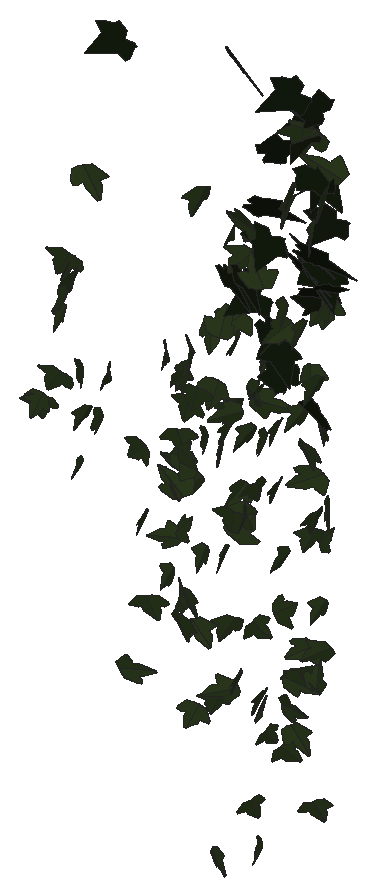
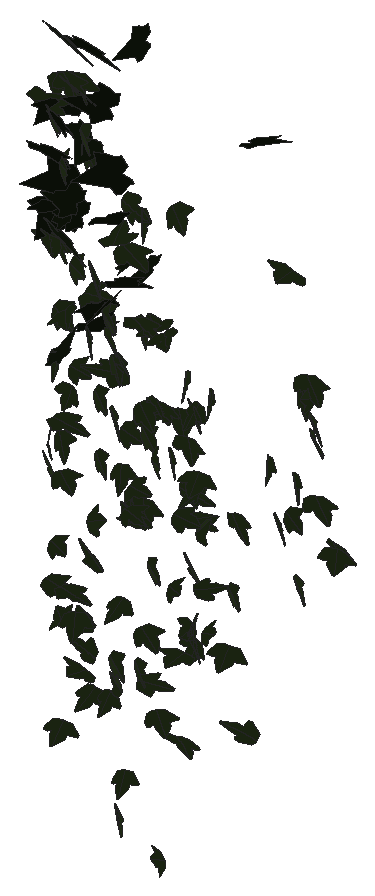
# SketchUp Ruby script. Lengths in inches.
U = 1.inch
M = Sketchup.active_model
def pt(a) = Geom::Point3d.new(a.map { |v| v * U })
def face(e, loops, mat)
  f = e.add_face(loops[0].map { |a| pt(a) })
  loops[1..].each { |l| e.add_face(l.map { |a| pt(a) }).erase! }
  f.material = f.back_material = mat if mat
  f
end
# faces: each face lists its corners as indices into pts; further lists are holes
def faces(e, pts, list, mat = nil) = list.each { |f| face(e, (f[0].is_a?(Array) ? f : [f]).map { |l| l.map { |i| pts[i] } }, mat) }
# xy, xz, yz: faces in a plane at the given z, y or x. An outline is a flat list of corners, or four numbers for a rectangle; further outlines are holes
def ring(l) = l.size == 4 ? [[l[0], l[1]], [l[2], l[1]], [l[2], l[3]], [l[0], l[3]]] : l.each_slice(2).to_a
def flat(e, list, mat, &to3) = list.each { |f| face(e, (f[0].is_a?(Array) ? f : [f]).map { |l| ring(l).map { |u, v| to3.(u, v) } }, mat) }
def xy(e, z, list, mat = nil) = flat(e, list, mat) { |x, y| [x, y, z] }
def xz(e, y, list, mat = nil) = flat(e, list, mat) { |x, z| [x, y, z] }
def yz(e, x, list, mat = nil) = flat(e, list, mat) { |y, z| [x, y, z] }
def lines(e, pts, list) = list.each { |a, b| e.add_line(pt(pts[a]), pt(pts[b])) }
# prism: a flat outline (further loops are holes) pulled along v
def prism(e, loops, v, mat = nil)
  f = face(e, loops, mat); d = Geom::Vector3d.new(v.map { |x| x * U })
  f.pushpull(f.normal.samedirection?(d) ? d.length : -d.length)
end
def box(e, o, s, mat = nil) = prism(e, [[o, [o[0] + s[0], o[1], o[2]], [o[0] + s[0], o[1] + s[1], o[2]], [o[0], o[1] + s[1], o[2]]]], [0, 0, s[2]], mat)
def at(x, y, z, deg = 0) = Geom::Transformation.translation(pt([x, y, z])) * Geom::Transformation.rotation(ORIGIN, Z_AXIS, deg.degrees)
def axes(o, x, y, z) = Geom::Transformation.new([*x, 0, *y, 0, *z, 0, *pt(o).to_a, 1])
def part(name) = M.definitions.add(name)
# library, detail: a bought-in or finely detailed component or shape, given as its bounding box
def library(name, o, s) = part(name).tap { |d| box(d.entities, o, s) }
def detail(e, o, s) = box(e.add_group.entities, o, s)
def put(e, d, t, mat = nil) = e.add_instance(d, t).tap { |i| i.material = mat if mat }
def group(e, t, mat = nil) = e.add_group.tap { |g| g.transformation = t; g.material = mat if mat }.entities
root = M.entities
M.materials.add("1026 AP 7946 SUNNY SIDE UP").color = [254, 231, 186]
M.materials.add("efeu1").color = [18, 25, 13]
M.materials.add("efeu2").color = [43, 57, 29]
c1 = part("ivyleaf_10")
p = [[0,0.5,-0.03],[-0.0625,2.02,-0.43],[-0.19,2.01,-0.46],[-0.54,1.05,-0.29],[-0.52,0.625,-0.18],[-0.83,0.76,-0.28],
  [-1.16,0.64,-0.33],[-1.15,0.33,-0.24],[-0.77,-0.39,0.02],[-0.3,-0.51,0.16],[0.04,-0.48,0.23],[-0.02,2.01,-0.4375],
  [-0.06,2.01,-0.43],[0.04,-0.49,0.23],[0.67,-0.49,0.14],[1.38,0.36,-0.2],[1.375,0.51,-0.24],[0.81,0.65,-0.19],
  [0.62,0.59,-0.15],[0.6,1.09,-0.28],[0.5,1.23,-0.31]]
faces(c1.entities,p,[[0,1,2,3,4,5,6,7,8,9,10],[11,12,0,13,14,15,16,17,18,19,20]],"efeu2")
c2 = part("ivyleaf_9")
p = [[1.54,2.16,1.25],[1.36,2.04,1.19],[-0.21,0.99,0.68],[-0.71,1.11,0.82],[-0.85,0.86,0.67],[-0.8,0.17,0.21],
  [-0.9,-0.01,0.1],[-0.67,-0.16,-0.02],[-0.08,-0.08,-0.05],[-0.03,-0.6,-0.4],[0.65,-0.88,-0.66],[0.83,-0.6,-0.49],
  [1.29,-0.42,-0.43],[1.8125,-0.07,-0.26],[1.21,0.44,0.15]]
faces(c2.entities,p,[[0,1,2,3,4,5,6,7,8,9,10,11,12,13,14]],"efeu1")
put(root,c1,axes([95.64,212.17,263.23],[0.16786,0.23551,-0.00023],[-0.02504,0.00892,0.26578],[0.36948,-0.10639,0.01811]),"1026 AP 7946 SUNNY SIDE UP")
put(root,c1,axes([91.38,212.24,264.06],[0.30214,0.04926,0.1328],[0.20568,0.0039,-0.20282],[-0.06785,0.2312,-0.02346]),"1026 AP 7946 SUNNY SIDE UP")
put(root,c1,axes([94.79,212.35,254.04],[-0.09675,-0.01931,0.21053],[-0.15756,-0.18349,-0.04999],[0.28189,-0.10919,0.04432]),"1026 AP 7946 SUNNY SIDE UP")
put(root,c1,axes([96.28,212.33,265.35],[0.14466,-0.21933,0.09608],[0.05974,-0.08655,-0.24552],[0.37074,0.09952,0.00207]),"1026 AP 7946 SUNNY SIDE UP")
put(root,c2,axes([94.92,212.24,267.83],[0.33388,-0.15464,-0.02679],[-0.04658,0.00193,-0.27011],[0.2419,0.21381,-0.01503]),"1026 AP 7946 SUNNY SIDE UP")
put(root,c1,axes([97.04,212.36,265.52],[0.15909,-0.19838,0.13997],[0.10649,-0.1192,-0.23005],[0.36382,0.12164,0.00613]),"1026 AP 7946 SUNNY SIDE UP")
put(root,c1,axes([91.3,212.34,258.85],[-0.00142,-0.18556,0.10339],[0.01134,-0.10138,-0.19163],[0.33232,0.00267,0.00698]),"1026 AP 7946 SUNNY SIDE UP")
put(root,c1,axes([96.17,212.29,254.15],[-0.07682,-0.00752,0.2101],[0.31914,-0.02411,0.04902],[0.03415,0.20836,0.01449]),"1026 AP 7946 SUNNY SIDE UP")
put(root,c1,axes([95.58,212.32,254.22],[0.0656,-0.21072,0.0622],[0.00929,-0.06157,-0.22157],[0.34507,0.04172,-0.00586]),"1026 AP 7946 SUNNY SIDE UP")
put(root,c1,axes([96.22,212.36,265.07],[0.0718,-0.22798,0.10513],[0.064,-0.09689,-0.23929],[0.38836,0.05812,0.02]),"1026 AP 7946 SUNNY SIDE UP")
put(root,c1,axes([96.48,212.39,262.46],[0.04991,-0.17184,0.15623],[0.07976,-0.14504,-0.17994],[0.35248,0.05715,0.0186]),"1026 AP 7946 SUNNY SIDE UP")
put(root,c1,axes([96.37,212.28,253.71],[0.23917,0.03312,0.14815],[0.2292,-0.00325,-0.15828],[-0.03431,0.20917,-0.02466]),"1026 AP 7946 SUNNY SIDE UP")
put(root,c1,axes([96,212.32,256.14],[0.21586,-0.11519,-0.15449],[0.1957,-0.08341,0.18369],[-0.22278,-0.18488,0.01166]),"1026 AP 7946 SUNNY SIDE UP")
put(root,c1,axes([93.7,212.25,255.21],[-0.29776,0.10063,-0.01107],[0.00201,-0.02162,-0.22023],[-0.15922,-0.18847,0.01792]),"1026 AP 7946 SUNNY SIDE UP")
put(root,c1,axes([95,212.25,261.7],[0.07048,-0.21323,-0.06226],[-0.03075,0.05638,-0.22402],[0.34662,0.04836,-0.00721]),"1026 AP 7946 SUNNY SIDE UP")
put(root,c1,axes([94.42,212.36,250.33],[-0.11791,0.07786,-0.17835],[0.15266,-0.14477,-0.11097],[-0.25723,-0.12161,0.0159]),"1026 AP 7946 SUNNY SIDE UP")
put(root,c1,axes([96.89,212.28,258.57],[-0.02156,-0.23029,-0.02042],[0.00928,0.01819,-0.23751],[0.36316,-0.01414,0.00486]),"1026 AP 7946 SUNNY SIDE UP")
put(root,c1,axes([92.38,212.22,253.67],[-0.11341,-0.01184,0.2055],[0.28023,0.09226,0.07254],[-0.14233,0.19107,-0.02091]),"1026 AP 7946 SUNNY SIDE UP")
put(root,c1,axes([92.9,212.25,255.34],[-0.27858,-0.11741,-0.0575],[0.08898,0.01404,-0.21801],[0.18354,-0.18502,0.01841]),"1026 AP 7946 SUNNY SIDE UP")
put(root,c2,axes([95.08,212.37,263.1],[0.1266,-0.2285,0.01316],[-0.003,-0.01558,-0.24957],[0.35996,0.08023,-0.00671]),"1026 AP 7946 SUNNY SIDE UP")
put(root,c2,axes([94.69,212.32,263.03],[0.21576,-0.19859,-0.01662],[-0.0192,0.0098,-0.24857],[0.31256,0.13769,-0.00379]),"1026 AP 7946 SUNNY SIDE UP")
put(root,c1,axes([95.73,212.35,261.75],[0.06974,-0.21548,0.05792],[0.01757,-0.05635,-0.22697],[0.35021,0.04574,-0.00014]),"1026 AP 7946 SUNNY SIDE UP")
put(root,c1,axes([96.84,212.4,261.38],[-0.00803,-0.21322,0.12062],[0.01681,-0.11841,-0.22007],[0.38304,0.00073,0.01219]),"1026 AP 7946 SUNNY SIDE UP")
put(root,c1,axes([96.91,212.25,252.32],[-0.21487,-0.13311,-0.07423],[0.08875,0.04416,-0.19612],[0.22022,-0.14767,0.00662]),"1026 AP 7946 SUNNY SIDE UP")
put(root,c1,axes([95.23,212.43,260.63],[-0.0278,0.00123,-0.2412],[0.18395,-0.20335,-0.01139],[-0.31892,-0.1174,0.01445]),"1026 AP 7946 SUNNY SIDE UP")
put(root,c1,axes([96.3,212.27,254.78],[0.01902,0.01261,0.21781],[0.31795,0.06211,-0.01537],[-0.09876,0.20239,-0.00755]),"1026 AP 7946 SUNNY SIDE UP")
put(root,c2,axes([96.67,212.25,264.18],[0.37162,-0.02784,0.12464],[0.19414,-0.02554,-0.23639],[0.062,0.2468,-0.00688]),"1026 AP 7946 SUNNY SIDE UP")
put(root,c2,axes([95.95,212.36,261.82],[-0.05006,-0.23005,-0.0786],[0.0228,0.07369,-0.23879],[0.37978,-0.03475,0.00398]),"1026 AP 7946 SUNNY SIDE UP")
put(root,c2,axes([96.17,212.29,261.21],[-0.2566,-0.17289,0.06578],[0.0597,0.05326,0.24507],[-0.28413,0.16733,-0.00792]),"1026 AP 7946 SUNNY SIDE UP")
put(root,c1,axes([95.58,212.22,250.92],[0.07459,-0.1589,-0.14756],[-0.07424,0.13437,-0.16997],[0.32712,0.06673,-0.00493]),"1026 AP 7946 SUNNY SIDE UP")
put(root,c1,axes([96.19,212.22,253.29],[-0.13961,-0.14649,-0.14868],[0.13973,0.11342,-0.17528],[0.29058,-0.12492,0.01286]),"1026 AP 7946 SUNNY SIDE UP")
put(root,c1,axes([93.61,212.28,257.95],[0.24893,0.08396,0.15275],[-0.24783,-0.00313,0.17573],[0.10009,-0.21656,0.05523]),"1026 AP 7946 SUNNY SIDE UP")
put(root,c1,axes([96.7,212.46,264.61],[0.08286,-0.1645,0.19208],[0.16923,-0.15775,-0.17478],[0.35367,0.11402,0.03863]),"1026 AP 7946 SUNNY SIDE UP")
put(root,c1,axes([94.34,212.35,261.72],[0.12731,0.21421,-0.0697],[-0.02628,-0.06727,-0.23617],[-0.35282,0.0823,-0.00756]),"1026 AP 7946 SUNNY SIDE UP")
put(root,c1,axes([94.04,212.39,264.5],[-0.06595,-0.23156,0.07293],[0.02,-0.07518,-0.24152],[0.38083,-0.03615,0.02531]),"1026 AP 7946 SUNNY SIDE UP")
put(root,c1,axes([94.9,212.3125,257.84],[-0.35593,-0.0086,0.0396],[-0.05881,-0.02441,-0.23234],[0.01969,-0.22831,0.022]),"1026 AP 7946 SUNNY SIDE UP")
put(root,c1,axes([90.66,212.34,259.39],[-0.29706,-0.02791,0.09692],[-0.13682,-0.04746,-0.19446],[0.07187,-0.20572,0.03042]),"1026 AP 7946 SUNNY SIDE UP")
put(root,c1,axes([90.67,212.4,260.77],[0.21533,-0.16354,0.05049],[0.03348,-0.04718,-0.21957],[0.26678,0.13792,-0.0132]),"1026 AP 7946 SUNNY SIDE UP")
put(root,c2,axes([97.02,212.27,267.32],[-0.23132,0.17871,0.11192],[-0.15107,0.05885,-0.23563],[-0.29117,-0.17251,0.03334]),"1026 AP 7946 SUNNY SIDE UP")
put(root,c1,axes([95.35,212.3,251.8],[-0.11303,-0.18466,-0.07817],[0.06774,0.06327,-0.2031],[0.30589,-0.08225,0.01609]),"1026 AP 7946 SUNNY SIDE UP")
put(root,c1,axes([94.95,212.38,254.35],[0.07566,-0.19636,0.01653],[-0.00087,-0.01779,-0.20832],[0.30993,0.04789,-0.00462]),"1026 AP 7946 SUNNY SIDE UP")
put(root,c1,axes([94.76,212.51,259.93],[-0.02153,-0.03243,0.23276],[-0.07883,-0.22058,-0.03701],[0.35044,-0.05161,0.00598]),"1026 AP 7946 SUNNY SIDE UP")
put(root,c1,axes([94.9,212.28,264.09],[0.06729,-0.20854,-0.13098],[-0.0055,0.12734,-0.21769],[0.38305,0.03847,0.01988]),"1026 AP 7946 SUNNY SIDE UP")
put(root,c1,axes([93.8,212.3125,258.52],[0.02249,-0.03548,-0.23672],[-0.33177,0.09425,-0.028],[0.15282,0.20983,-0.02594]),"1026 AP 7946 SUNNY SIDE UP")
put(root,c2,axes([95.84,212.2,266.06],[0.07736,0.04128,0.25866],[0.35028,0.1161,-0.06402],[-0.1926,0.22774,-0.01253]),"1026 AP 7946 SUNNY SIDE UP")
put(root,c2,axes([96.35,212.44,267.41],[-0.41475,0.02382,0.02148],[-0.03716,-0.02186,-0.26187],[-0.03714,-0.24414,0.02207]),"1026 AP 7946 SUNNY SIDE UP")
put(root,c2,axes([96.28,212.15,265.19],[0.14187,0.19093,0.16969],[0.04759,0.1563,-0.21868],[-0.41583,0.08303,0.03286]),"1026 AP 7946 SUNNY SIDE UP")
put(root,c1,axes([90.74,212.37,261.12],[0.15591,-0.19237,-0.04358],[-0.04719,0.03081,-0.22241],[0.30572,0.10286,-0.01211]),"1026 AP 7946 SUNNY SIDE UP")
put(root,c1,axes([91.2,212.31,259.69],[0.16273,-0.14698,-0.12449],[-0.04758,0.12216,-0.18031],[0.29455,0.10094,0.03965]),"1026 AP 7946 SUNNY SIDE UP")
put(root,c1,axes([95.47,212.34,253.6875],[0.13447,-0.17319,0.06351],[-0.02957,0.06048,0.1991],[-0.28807,-0.08705,0.0092]),"1026 AP 7946 SUNNY SIDE UP")
put(root,c2,axes([95.48,212.26,264.78],[0.31812,0.06339,0.14339],[0.21808,0.01984,-0.21743],[-0.10015,0.24456,-0.01799]),"1026 AP 7946 SUNNY SIDE UP")
put(root,c1,axes([90.83,212.39,261.96],[-0.31617,-0.02862,0.09718],[-0.13917,-0.0428,-0.20761],[0.06882,-0.21801,0.02665]),"1026 AP 7946 SUNNY SIDE UP")
put(root,c2,axes([95.3,212.55,262.63],[-0.28259,-0.12882,0.10334],[-0.09704,-0.08567,-0.2261],[0.23845,-0.18753,0.03046]),"1026 AP 7946 SUNNY SIDE UP")
put(root,c1,axes([93.96,212.39,260.15],[-0.31971,-0.05305,0.05034],[-0.06597,-0.033,-0.21561],[0.09265,-0.20657,0.0202]),"1026 AP 7946 SUNNY SIDE UP")
put(root,c2,axes([96.93,212.24,263.48],[0.29213,0.16607,0.04339],[0.04386,0.02847,-0.25562],[-0.28599,0.174,0.00512]),"1026 AP 7946 SUNNY SIDE UP")
put(root,c1,axes([90.1,212.43,258.65],[0.29324,-0.08452,-0.00301],[-0.01427,-0.01413,-0.21032],[0.13219,0.18597,-0.01603]),"1026 AP 7946 SUNNY SIDE UP")
put(root,c1,axes([90.9375,212.39,261.63],[-0.01055,-0.22128,-0.0399],[0.00988,0.03729,-0.22779],[0.35276,-0.00766,0.00519]),"1026 AP 7946 SUNNY SIDE UP")
put(root,c1,axes([91.84,212.31,259.84],[0.04001,-0.16585,-0.14488],[0.00064,0.14068,-0.17117],[0.34095,0.0192,0.01732]),"1026 AP 7946 SUNNY SIDE UP")
put(root,c1,axes([94.58,212.29,261.74],[0.18778,0.18076,-0.1112],[0.06795,0.1016,0.22303],[0.32484,-0.12575,0.01763]),"1026 AP 7946 SUNNY SIDE UP")
put(root,c1,axes([95.25,212.29,264.21],[0.0552,0.00663,-0.2553],[-0.28931,0.1685,-0.02121],[0.26134,0.18513,0.03044]),"1026 AP 7946 SUNNY SIDE UP")
put(root,c1,axes([93.65,212.4375,255.65],[-0.21419,0.11574,-0.11703],[0.11714,-0.08807,-0.18393],[-0.22732,-0.15444,0.01548]),"1026 AP 7946 SUNNY SIDE UP")
put(root,c1,axes([95.91,212.57,257.22],[0.04529,-0.06617,0.21828],[0.08701,-0.20517,-0.07482],[0.3386,0.06157,-0.00997]),"1026 AP 7946 SUNNY SIDE UP")
put(root,c1,axes([93.68,212.37,255.54],[-0.13095,0.19429,-0.02789],[-0.01486,0.0266,0.21791],[0.30834,0.08379,-0.00134]),"1026 AP 7946 SUNNY SIDE UP")
put(root,c2,axes([96.28,212.49,263.69],[0.22763,-0.14634,0.14454],[0.14506,-0.10711,-0.21253],[0.28488,0.17147,-0.00727]),"1026 AP 7946 SUNNY SIDE UP")
put(root,c1,axes([93.61,212.41,260.43],[0.2093,-0.17793,-0.04358],[-0.03191,0.03638,-0.22863],[0.28543,0.13454,0.0064]),"1026 AP 7946 SUNNY SIDE UP")
put(root,c1,axes([93.23,212.32,260.79],[0.0986,-0.16889,-0.14244],[0.01462,0.14484,-0.17831],[0.34194,0.04251,0.0487]),"1026 AP 7946 SUNNY SIDE UP")
put(root,c1,axes([95.69,212.33,253.42],[-0.08721,-0.15189,-0.12977],[0.07387,0.116,-0.16586],[0.30047,-0.07261,0.00312]),"1026 AP 7946 SUNNY SIDE UP")
put(root,c1,axes([95.49,212.37,260.52],[-0.03274,-0.03439,-0.24112],[0.369,0.0251,-0.02518],[0.04451,-0.23344,0.0314]),"1026 AP 7946 SUNNY SIDE UP")
put(root,c1,axes([94.92,212.37,257.46],[0.31731,-0.02251,-0.10351],[0.1611,0.02487,0.20666],[-0.01401,-0.224,0.03201]),"1026 AP 7946 SUNNY SIDE UP")
put(root,c2,axes([96.92,212.48,263.75],[-0.09535,-0.22844,-0.10259],[0.04478,0.09412,-0.24291],[0.38846,-0.06692,0.00282]),"1026 AP 7946 SUNNY SIDE UP")
put(root,c1,axes([93.46,212.35,257.79],[-0.1547,0.1685,-0.12008],[-0.10686,0.09627,0.20137],[0.30483,0.11926,0.00965]),"1026 AP 7946 SUNNY SIDE UP")
put(root,c1,axes([91.07,212.43,257.55],[0.10037,-0.18939,-0.03867],[-0.03727,0.03042,-0.20531],[0.30097,0.06693,-0.01253]),"1026 AP 7946 SUNNY SIDE UP")
put(root,c1,axes([95.47,212.42,260.79],[0.01908,-0.21781,-0.04329],[-0.01725,0.0402,-0.22433],[0.34801,0.01393,-0.00874]),"1026 AP 7946 SUNNY SIDE UP")
put(root,c2,axes([95.55,212.59,263.95],[-0.18465,-0.21554,0.04218],[-0.01171,-0.04388,-0.2527],[0.34515,-0.1168,0.01399]),"1026 AP 7946 SUNNY SIDE UP")
put(root,c1,axes([96.91,212.53,255.55],[-0.13531,-0.09053,0.16456],[-0.13366,-0.13735,-0.12777],[0.25669,-0.11924,0.02021]),"1026 AP 7946 SUNNY SIDE UP")
put(root,c2,axes([96.5,212.52,263.6875],[0.22457,-0.19906,0.05326],[0.02577,-0.0531,-0.25207],[0.32281,0.14272,-0.01693]),"1026 AP 7946 SUNNY SIDE UP")
put(root,c1,axes([96.57,212.5,255.49],[0.22524,0.02747,-0.15019],[-0.21435,-0.0561,-0.14905],[-0.09261,0.19665,-0.02027]),"1026 AP 7946 SUNNY SIDE UP")
put(root,c2,axes([96.8,212.43,265.9],[-0.05145,-0.18391,-0.1877],[0.09361,0.17231,-0.19028],[0.39498,-0.0648,0.02065]),"1026 AP 7946 SUNNY SIDE UP")
put(root,c1,axes([93.25,212.58,256.6875],[-0.01149,0.0473,0.20817],[-0.12012,-0.18832,0.04153],[0.30297,-0.07287,0.02436]),"1026 AP 7946 SUNNY SIDE UP")
put(root,c1,axes([91.55,212.43,258.73],[0.14154,-0.17323,-0.08362],[-0.06557,0.06867,-0.20065],[0.29291,0.09908,-0.00451]),"1026 AP 7946 SUNNY SIDE UP")
put(root,c1,axes([94.13,212.4,259.23],[0.13757,-0.15834,-0.11357],[-0.04642,0.10765,-0.1843],[0.29899,0.08957,0.02364]),"1026 AP 7946 SUNNY SIDE UP")
put(root,c1,axes([95.96,212.58,262.17],[0.13284,0.10233,-0.21171],[-0.18225,-0.17072,-0.13728],[-0.31254,0.14305,-0.00993]),"1026 AP 7946 SUNNY SIDE UP")
put(root,c1,axes([95.5625,212.5625,261.78],[0.17412,-0.18307,0.10864],[0.06955,-0.09754,-0.22067],[0.32568,0.1187,-0.01096]),"1026 AP 7946 SUNNY SIDE UP")
put(root,c1,axes([93.82,212.5,253.2],[0.31342,-0.01718,-0.03212],[-0.05114,-0.01715,-0.20521],[0.02243,0.201,-0.01907]),"1026 AP 7946 SUNNY SIDE UP")
put(root,c1,axes([93.76,212.6,258.09],[-0.0593,-0.1166,0.18174],[-0.04806,-0.17498,-0.12644],[0.32989,-0.04645,0.01425]),"1026 AP 7946 SUNNY SIDE UP")
put(root,c1,axes([96.28,212.61,260.43],[-0.03123,-0.133,0.17821],[0.02226,-0.17487,-0.13726],[0.34332,-0.00076,0.02511]),"1026 AP 7946 SUNNY SIDE UP")
put(root,c2,axes([97.13,212.56,264.91],[-0.37037,-0.05513,-0.02284],[0.04308,-0.01672,-0.23997],[0.09014,-0.21852,0.02085]),"1026 AP 7946 SUNNY SIDE UP")
put(root,c1,axes([96.92,212.5,257.88],[0.16139,-0.16764,-0.06153],[0.07328,-0.04009,0.20142],[-0.26955,-0.11128,0.01792]),"1026 AP 7946 SUNNY SIDE UP")
put(root,c1,axes([96.89,212.5,263.02],[0.2937,-0.16846,-0.02784],[-0.04619,0.00628,-0.25863],[0.26404,0.18849,-0.01428]),"1026 AP 7946 SUNNY SIDE UP")
put(root,c1,axes([96.62,212.5,261.48],[0.08326,0.23008,-0.07252],[-0.02638,-0.06971,-0.24363],[-0.37801,0.05554,0.00103]),"1026 AP 7946 SUNNY SIDE UP")
put(root,c1,axes([95.1,212.35,257.87],[0.03734,-0.13584,-0.18941],[-0.01955,0.18304,-0.14049],[0.35795,0.02417,0.01208]),"1026 AP 7946 SUNNY SIDE UP")
put(root,c1,axes([94.9,212.58,258.33],[0.07669,0.13903,-0.17447],[-0.13554,-0.14821,-0.15109],[-0.31781,0.09676,0.02233]),"1026 AP 7946 SUNNY SIDE UP")
put(root,c1,axes([90.8,212.34,261.58],[0.06127,-0.095,0.20249],[-0.11145,0.18392,0.10684],[-0.32548,-0.08086,0.00154]),"1026 AP 7946 SUNNY SIDE UP")
put(root,c1,axes([95.49,212.46,259.65],[0.14123,-0.20116,-0.07303],[-0.04172,0.06453,-0.22657],[0.33217,0.09363,0.00259]),"1026 AP 7946 SUNNY SIDE UP")
put(root,c1,axes([95.77,212.56,260.01],[0.05658,-0.20645,0.06167],[0.02412,-0.05927,-0.21618],[0.33765,0.03883,0.00511]),"1026 AP 7946 SUNNY SIDE UP")
put(root,c1,axes([96.4,212.47,254.92],[-0.20076,-0.18349,-0.03709],[0.04871,0.02096,-0.22976],[0.28964,-0.13071,0.01293]),"1026 AP 7946 SUNNY SIDE UP")
put(root,c2,axes([96.87,212.57,265.74],[-0.31692,0.01599,-0.14733],[0.22918,-0.03239,-0.20025],[-0.05436,-0.22978,0.01469]),"1026 AP 7946 SUNNY SIDE UP")
put(root,c1,axes([96.78,212.61,256.45],[-0.04925,-0.14817,0.1373],[0.04099,-0.13762,-0.15117],[0.31157,-0.00531,0.04159]),"1026 AP 7946 SUNNY SIDE UP")
put(root,c1,axes([96.63,212.56,257.96],[-0.15695,-0.16096,0.0779],[-0.02347,-0.07986,-0.19355],[0.27926,-0.09717,0.02752]),"1026 AP 7946 SUNNY SIDE UP")
put(root,c1,axes([94.69,212.56,260.09],[-0.08489,-0.21346,0.06137],[-0.01642,-0.06005,-0.22713],[0.3486,-0.05481,0.00425]),"1026 AP 7946 SUNNY SIDE UP")
put(root,c1,axes([94.26,212.54,260.32],[0.34088,-0.06468,0.0128],[0.01021,-0.02279,-0.23229],[0.10316,0.21597,-0.01929]),"1026 AP 7946 SUNNY SIDE UP")
put(root,c1,axes([94.6,212.57,259.6],[0.04454,-0.21504,0.06724],[0.01667,-0.06567,-0.22382],[0.35353,0.03019,0.00208]),"1026 AP 7946 SUNNY SIDE UP")
put(root,c1,axes([94.34,212.63,259.08],[0.10505,-0.11865,0.17988],[0.15439,-0.14546,-0.14084],[0.29485,0.11844,0.00966]),"1026 AP 7946 SUNNY SIDE UP")
put(root,c1,axes([95.96,212.49,262.61],[0.19556,-0.20396,-0.06025],[-0.03896,0.05202,-0.24573],[0.33085,0.12669,0.00668]),"1026 AP 7946 SUNNY SIDE UP")
put(root,c1,axes([95.34,212.42,255.59],[-0.10034,-0.16768,-0.13666],[0.14078,0.10369,-0.18009],[0.30427,-0.10327,0.03826]),"1026 AP 7946 SUNNY SIDE UP")
put(root,c1,axes([96.42,212.5,266.59],[-0.33181,-0.13474,0.00843],[0.00321,-0.01978,-0.25739],[0.21231,-0.21028,0.01706]),"1026 AP 7946 SUNNY SIDE UP")
put(root,c1,axes([92.52,212.46,258.42],[0.25192,-0.07839,-0.11845],[-0.13091,0.08568,-0.17988],[0.17461,0.17733,0.03603]),"1026 AP 7946 SUNNY SIDE UP")
put(root,c1,axes([96.54,212.48,259.8],[-0.28764,0.11151,-0.01354],[0.00682,-0.0193,-0.22034],[-0.17654,-0.18243,0.01355]),"1026 AP 7946 SUNNY SIDE UP")
put(root,c2,axes([96.68,212.66,260.54],[0.17901,-0.21113,-0.05592],[0.05395,-0.04175,0.24665],[-0.33804,-0.11847,0.00975]),"1026 AP 7946 SUNNY SIDE UP")
put(root,c1,axes([95.03,212.59,263.4],[-0.25649,-0.09589,0.14204],[-0.12209,-0.12818,-0.18648],[0.23495,-0.17129,0.05816]),"1026 AP 7946 SUNNY SIDE UP")
put(root,c1,axes([97.14,212.54,265.89],[0.17007,0.09072,0.21825],[-0.30793,-0.09482,0.14011],[0.21743,-0.20525,0.02771]),"1026 AP 7946 SUNNY SIDE UP")
put(root,c2,axes([96.89,212.41,263.15],[-0.19216,0.20583,0.08984],[-0.09577,0.06359,-0.24548],[-0.33746,-0.13526,0.0185]),"1026 AP 7946 SUNNY SIDE UP")
put(root,c2,axes([95.54,212.5,262.1],[0.15673,-0.19114,-0.11411],[-0.07625,0.0984,-0.22149],[0.33802,0.11082,0.00295]),"1026 AP 7946 SUNNY SIDE UP")
put(root,c1,axes([95.48,212.6,261.35],[0.17853,-0.17145,0.09098],[0.05718,-0.08275,-0.21183],[0.29852,0.11838,-0.01384]),"1026 AP 7946 SUNNY SIDE UP")
put(root,c1,axes([93.42,212.56,256.9],[0.17518,-0.15247,-0.09466],[0.10628,-0.06295,0.19349],[-0.25819,-0.12936,0.01543]),"1026 AP 7946 SUNNY SIDE UP")
put(root,c1,axes([93.43,212.5,259.02],[-0.25822,-0.11928,-0.05043],[0.08759,0.00466,-0.20705],[0.18239,-0.17111,0.02803]),"1026 AP 7946 SUNNY SIDE UP")
put(root,c1,axes([93.51,212.35,258.64],[0.02374,0.1088,0.20314],[0.00014,0.19701,-0.11119],[-0.35328,0.00739,0.01361]),"1026 AP 7946 SUNNY SIDE UP")
put(root,c1,axes([93.76,212.39,261],[0.12218,-0.12267,-0.18371],[-0.00674,0.18787,-0.1345],[0.33937,0.0479,0.06347]),"1026 AP 7946 SUNNY SIDE UP")
put(root,c1,axes([93.59,212.45,255.45],[0.10219,-0.14694,-0.13825],[-0.10712,0.11528,-0.16438],[0.29306,0.09338,-0.01188]),"1026 AP 7946 SUNNY SIDE UP")
put(root,c1,axes([93.83,212.48,255.03],[0.22335,0.11716,0.10668],[0.14472,0.04935,-0.1885],[-0.19791,0.16831,-0.01744]),"1026 AP 7946 SUNNY SIDE UP")
put(root,c1,axes([93.08,212.66,255.83],[-0.03472,-0.08046,0.19046],[0.10555,-0.17877,-0.07276],[0.29965,0.05365,0.0477]),"1026 AP 7946 SUNNY SIDE UP")
put(root,c1,axes([93.51,212.41,260.43],[-0.05138,-0.15154,-0.16999],[0.08912,0.15484,-0.15798],[0.33978,-0.06353,0.01573]),"1026 AP 7946 SUNNY SIDE UP")
put(root,c1,axes([96.08,212.47,261.2],[0.13136,-0.18099,-0.10832],[-0.03733,0.10318,-0.20379],[0.32618,0.0847,0.0203]),"1026 AP 7946 SUNNY SIDE UP")
put(root,c1,axes([96.65,212.59,259.1875],[0.22153,0.03859,-0.18526],[-0.26344,-0.0672,-0.15029],[-0.12014,0.21852,-0.01206]),"1026 AP 7946 SUNNY SIDE UP")
put(root,c1,axes([96.875,212.66,258.59],[0.07575,-0.0985,0.20896],[0.21923,-0.15071,-0.11009],[0.27965,0.14483,0.02971]),"1026 AP 7946 SUNNY SIDE UP")
put(root,c1,axes([92.53,212.58,256.9],[0.09186,-0.19049,0.03975],[0.01331,-0.03889,-0.20547],[0.30567,0.05894,-0.003]),"1026 AP 7946 SUNNY SIDE UP")
put(root,c1,axes([96.61,212.57,266.56],[-0.31213,-0.02729,0.16107],[-0.2247,-0.09042,-0.19156],[0.13111,-0.21994,0.05513]),"1026 AP 7946 SUNNY SIDE UP")
put(root,c1,axes([94.92,212.66,257.81],[-0.13748,-0.12958,0.15514],[-0.00637,-0.16407,-0.1481],[0.31321,-0.06022,0.06508]),"1026 AP 7946 SUNNY SIDE UP")
put(root,c1,axes([90.05,212.53,258.56],[-0.30049,-0.0687,-0.00543],[0.01673,-0.01522,-0.20848],[0.10699,-0.19056,0.01735]),"1026 AP 7946 SUNNY SIDE UP")
put(root,c2,axes([96.3,212.62,264.01],[0.20442,-0.15768,0.14002],[0.14813,-0.09952,-0.21096],[0.29294,0.16036,0.00896]),"1026 AP 7946 SUNNY SIDE UP")
put(root,c1,axes([94.77,212.59,261.96],[0.31166,0.01726,-0.11654],[-0.1707,-0.04384,-0.20291],[-0.05742,0.22402,-0.02936]),"1026 AP 7946 SUNNY SIDE UP")
put(root,c2,axes([91.89,212.72,266.92],[-0.26515,-0.10959,0.14893],[-0.13582,-0.12599,-0.20206],[0.25172,-0.18341,0.04785]),"1026 AP 7946 SUNNY SIDE UP")
put(root,c1,axes([95.26,212.5,258.54],[-0.0864,-0.20643,-0.07366],[0.03296,0.06719,-0.21966],[0.34133,-0.05874,0.00256]),"1026 AP 7946 SUNNY SIDE UP")
put(root,c1,axes([94.99,212.68,259.55],[-0.00852,-0.15513,0.16935],[0.01591,-0.16531,-0.16049],[0.35606,0.00367,0.01122]),"1026 AP 7946 SUNNY SIDE UP")
put(root,c1,axes([96.78,212.41,254.78],[0.05954,0.17995,-0.1419],[0.02752,0.13795,0.19002],[0.35625,-0.04073,0.00904]),"1026 AP 7946 SUNNY SIDE UP")
put(root,c1,axes([93.625,212.55,259.73],[-0.32043,0.03115,0.05139],[-0.08634,-0.03811,-0.20755],[-0.03244,-0.20626,0.04483]),"1026 AP 7946 SUNNY SIDE UP")
put(root,c1,axes([94.6,212.62,255.31],[-0.14795,-0.1714,0.09088],[-0.03732,-0.0882,-0.20092],[0.30151,-0.09502,0.01972]),"1026 AP 7946 SUNNY SIDE UP")
put(root,c1,axes([94.43,212.63,256.77],[0.1245,-0.17729,0.08356],[0.04362,-0.07751,-0.20039],[0.30411,0.0837,-0.00547]),"1026 AP 7946 SUNNY SIDE UP")
put(root,c1,axes([96.84,212.51,260.4],[-0.21252,0.16762,0.03542],[-0.05956,0.01219,-0.22064],[-0.26208,-0.13869,0.02142]),"1026 AP 7946 SUNNY SIDE UP")
put(root,c2,axes([96.36,212.68,266.59],[-0.32208,-0.04727,-0.14214],[0.22859,-0.05342,-0.20419],[0.01251,-0.24097,0.07162]),"1026 AP 7946 SUNNY SIDE UP")
put(root,c1,axes([96.87,212.6,263.03],[0.37346,-0.01252,0.04252],[0.06275,-0.02493,-0.24407],[0.02602,0.23979,-0.02174]),"1026 AP 7946 SUNNY SIDE UP")
put(root,c1,axes([93.87,212.6875,256.55],[-0.03907,-0.13624,0.15748],[0.10506,-0.1517,-0.12834],[0.30531,0.03477,0.06431]),"1026 AP 7946 SUNNY SIDE UP")
put(root,c1,axes([95.73,212.59,258.69],[0.05625,-0.20621,0.0145],[0.00003,-0.01547,-0.21568],[0.32513,0.03568,-0.00249]),"1026 AP 7946 SUNNY SIDE UP")
put(root,c1,axes([94.29,212.6,253.6],[-0.20446,-0.1467,0.05056],[-0.03277,-0.04801,-0.20158],[0.24145,-0.13075,0.01546]),"1026 AP 7946 SUNNY SIDE UP")
